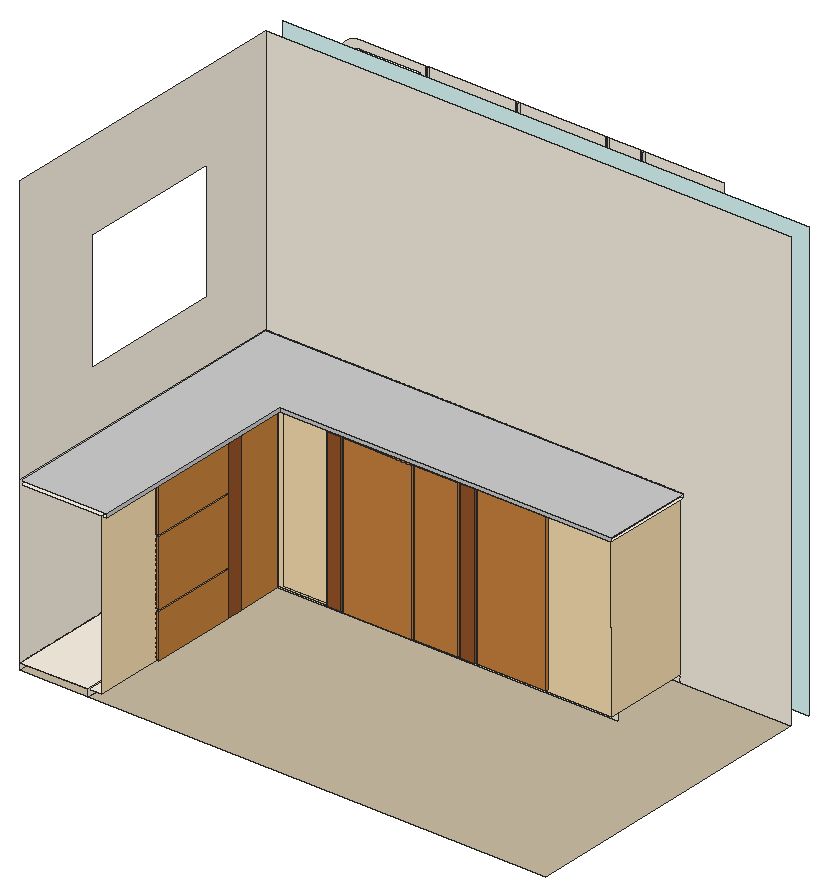
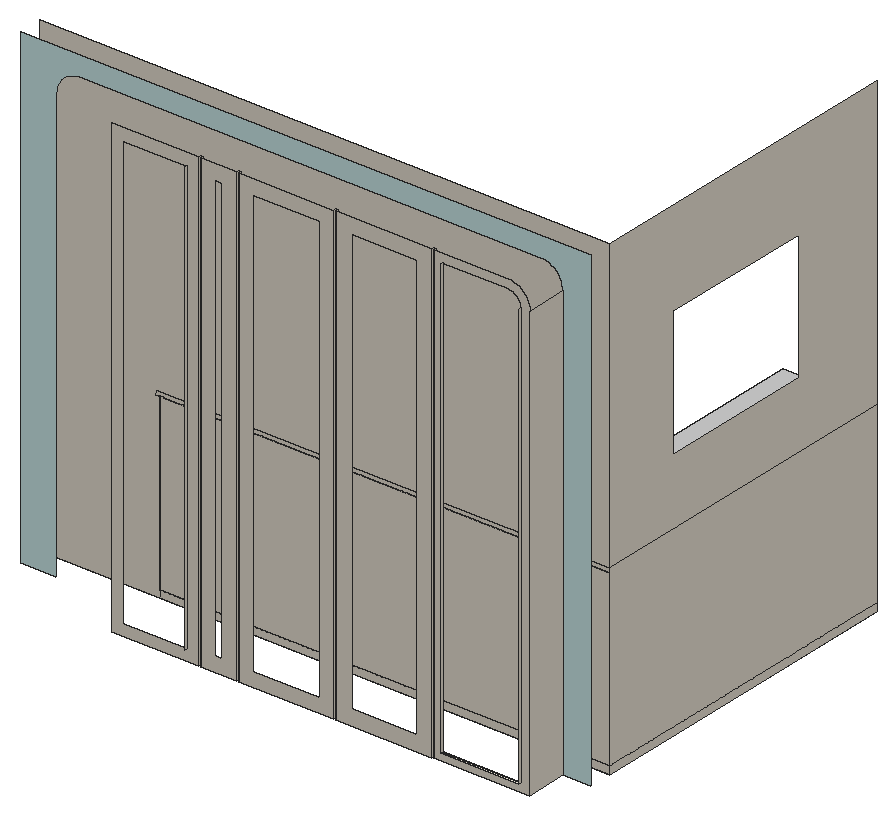
# SketchUp Ruby script. Lengths in inches.
U = 1.inch
M = Sketchup.active_model
def pt(a) = Geom::Point3d.new(a.map { |v| v * U })
def face(e, loops, mat)
  f = e.add_face(loops[0].map { |a| pt(a) })
  loops[1..].each { |l| e.add_face(l.map { |a| pt(a) }).erase! }
  f.material = f.back_material = mat if mat
  f
end
# faces: each face lists its corners as indices into pts; further lists are holes
def faces(e, pts, list, mat = nil) = list.each { |f| face(e, (f[0].is_a?(Array) ? f : [f]).map { |l| l.map { |i| pts[i] } }, mat) }
# xy, xz, yz: faces in a plane at the given z, y or x. An outline is a flat list of corners, or four numbers for a rectangle; further outlines are holes
def ring(l) = l.size == 4 ? [[l[0], l[1]], [l[2], l[1]], [l[2], l[3]], [l[0], l[3]]] : l.each_slice(2).to_a
def flat(e, list, mat, &to3) = list.each { |f| face(e, (f[0].is_a?(Array) ? f : [f]).map { |l| ring(l).map { |u, v| to3.(u, v) } }, mat) }
def xy(e, z, list, mat = nil) = flat(e, list, mat) { |x, y| [x, y, z] }
def xz(e, y, list, mat = nil) = flat(e, list, mat) { |x, z| [x, y, z] }
def yz(e, x, list, mat = nil) = flat(e, list, mat) { |y, z| [x, y, z] }
def lines(e, pts, list) = list.each { |a, b| e.add_line(pt(pts[a]), pt(pts[b])) }
# prism: a flat outline (further loops are holes) pulled along v
def prism(e, loops, v, mat = nil)
  f = face(e, loops, mat); d = Geom::Vector3d.new(v.map { |x| x * U })
  f.pushpull(f.normal.samedirection?(d) ? d.length : -d.length)
end
def box(e, o, s, mat = nil) = prism(e, [[o, [o[0] + s[0], o[1], o[2]], [o[0] + s[0], o[1] + s[1], o[2]], [o[0], o[1] + s[1], o[2]]]], [0, 0, s[2]], mat)
def at(x, y, z, deg = 0) = Geom::Transformation.translation(pt([x, y, z])) * Geom::Transformation.rotation(ORIGIN, Z_AXIS, deg.degrees)
def axes(o, x, y, z) = Geom::Transformation.new([*x, 0, *y, 0, *z, 0, *pt(o).to_a, 1])
def part(name) = M.definitions.add(name)
# library, detail: a bought-in or finely detailed component or shape, given as its bounding box
def library(name, o, s) = part(name).tap { |d| box(d.entities, o, s) }
def detail(e, o, s) = box(e.add_group.entities, o, s)
def put(e, d, t, mat = nil) = e.add_instance(d, t).tap { |i| i.material = mat if mat }
def group(e, t, mat = nil) = e.add_group.tap { |g| g.transformation = t; g.material = mat if mat }.entities
root = M.entities
M.materials.add("[0030_OldLace]").color = [253, 245, 230]
M.materials.add("[0032_Moccasin]").color = [255, 228, 181]
M.materials.add("[0040_Peru]").color = [205, 133, 63]
M.materials.add("[0090_LightCyan]").color = [224, 255, 255]
M.materials.add("[Carrera Marble]").color = [207, 207, 207]
M.materials.add("[Concrete Tile]").color = [203, 190, 164]
M.materials.add("[Wood Cherry Original]").color = [152, 86, 42]
xy(root,1.9375,[[9,301.46,9,385.46,122.59,385.46,122.59,361.96,31.28,361.96,31.28,301.46]],"[0030_OldLace]")
xy(root,2.2,[[18.24,402.03,37.94,402.71]],"[0030_OldLace]")
xy(root,2.4375,[[31.28,319.96,32.22,343.46],[31.28,343.93,32.22,347.96],[31.28,348.43,32.22,360.46],[49.79,360.87,49.78,361.93,68.78,361.96,68.79,360.9],[45.29,360.99,45.28,361.93,49.28,361.96,49.29,361.03],
  [69.29,360.99,69.28,361.93,81.28,361.96,81.29,361.03],[81.79,361.12,81.78,361.93,85.78,361.96,85.79,361.15],[86.29,361.24,86.28,361.93,105.28,361.96,105.29,361.28]],"[0030_OldLace]")
xy(root,14.4375,[[31.28,319.96,32.22,343.46]],"[0040_Peru]")
xy(root,14.9375,[[31.28,319.96,32.22,343.45]],"[0030_OldLace]")
xy(root,32.6875,[[31.28,319.96,32.22,343.45]],"[0040_Peru]")
xy(root,33.1875,[[31.28,319.96,32.22,343.4375]],"[0030_OldLace]")
xy(root,45.1875,[[31.28,319.96,32.22,343.4375],[31.28,348.43,32.22,360.46],[49.79,360.87,68.79,360.9,68.78,361.96,49.78,361.93],[69.29,360.99,81.29,361.03,81.28,361.96,69.28,361.93],[86.29,361.24,105.29,361.28,105.28,361.96,86.28,361.93]],"[0040_Peru]")
xy(root,45.1875,[[31.28,343.93,32.22,347.96],[45.29,360.99,49.29,361.03,49.28,361.96,45.28,361.93],[81.79,361.12,85.79,361.15,85.78,361.96,81.78,361.93]],"[Wood Cherry Original]")
xy(root,45.6875,[[9,301.46,9,385.46,123.52,385.46,123.52,360.6875,32.64,360.6875,32.64,301.46]],"[0030_OldLace]")
xy(root,46.625,[[9,301.46,32.64,301.46,32.64,360.6875,123.52,360.6875,123.52,385.46,9,385.46]],"[Carrera Marble]")
xz(root,319.96,[[31.28,2.4375,32.22,14.4375],[31.28,14.9375,32.22,32.6875],[31.28,33.1875,32.22,45.1875]],"[0040_Peru]")
xz(root,343.4375,[[31.28,33.1875,32.22,45.1875]],"[0030_OldLace]")
xz(root,343.45,[[31.28,14.9375,32.22,32.6875]],"[0030_OldLace]")
xz(root,343.46,[[31.28,2.4375,32.22,14.4375]],"[0030_OldLace]")
xz(root,343.93,[[31.28,2.4375,32.22,45.1875]],"[Wood Cherry Original]")
xz(root,347.96,[[31.28,2.4375,32.22,45.1875]],"[Wood Cherry Original]")
xz(root,348.43,[[31.28,2.4375,32.22,45.1875]],"[0040_Peru]")
xz(root,360.46,[[31.28,2.4375,32.22,45.1875]],"[0030_OldLace]")
xz(root,360.6875,[[32.64,45.6875,123.52,46.625]],"[Carrera Marble]")
xz(root,385.46,[[122.59,0,153,0,153,120,9,120,9,46.625,123.52,46.625,123.52,45.6875,122.59,45.6875],[9,0,122.59,1.9375],[9,1.9375,122.59,45.6875],[9,45.6875,123.52,46.625]],"[0030_OldLace]")
xz(root,391.46,[[9,0,9,120,153,120,153,0,143.9375,0,143.9375,108.93,143.89,109.72,143.73,110.5,143.48,111.25,143.125,111.96,142.68,112.625,142.16,113.22,141.5625,113.74,140.9,114.1875,140.1875,114.54,139.44,114.79,138.66,114.95,137.86,115,21.59,115,20.87,114.95,20.16,114.8125,19.47,114.58,18.82,114.26,18.22,113.85,17.67,113.375,17.19,112.83,16.79,112.23,16.47,111.58,16.24,110.89,16.1,110.18,16.05,109.45,16.05,0]],"[0090_LightCyan]")
xz(root,401.46,[[40.14,0,40.64,115],[64.9,0,65.38,115],[89.38,0,89.9375,115],[99.07,0,99.5625,115]],"[0030_OldLace]")
xz(root,402.03,[[[16.05,0,16.05,109.45,16.1,110.18,16.24,110.89,16.47,111.58,16.79,112.23,17.19,112.83,17.67,113.375,18.22,113.85,18.82,114.26,19.47,114.58,20.16,114.8125,20.87,114.95,21.59,115,40.14,115,40.14,0],[18.24,2.2,37.94,2.2,37.94,112.8,21.59,112.8,21.16,112.78,20.73,112.69,20.3125,112.55,19.92,112.36,19.55,112.11,19.22,111.82,18.9375,111.49,18.69,111.13,18.5,110.74,18.36,110.32,18.27,109.89,18.24,109.45]],[[40.64,0,64.9,115],[44.51,3.87,61.02,111.13]],[[65.38,0,89.38,115],[68.98,3.6,85.78,111.4]],[[89.9375,0,99.07,115],[93.66,3.73,95.34,111.27]],[[99.5625,0,121.45,115],[102.43,2.87,118.59,112.13]]],"[0030_OldLace]")
yz(root,9,[[301.46,0,385.46,1.9375],[301.46,1.9375,385.46,46.625],[[301.46,46.625,385.46,120],[326.03,63.5,365.53,96]]],"[0030_OldLace]")
yz(root,16.05,[[391.46,0,402.03,109.45]],"[0030_OldLace]")
yz(root,18.24,[[402.03,2.2,402.71,109.45]],"[0030_OldLace]")
yz(root,31.28,[[319.96,2.4375,343.46,14.4375],[343.93,2.4375,347.96,45.1875],[348.43,2.4375,360.46,45.1875],[319.96,14.9375,343.45,32.6875],[319.96,33.1875,343.4375,45.1875]],"[0030_OldLace]")
yz(root,32.22,[[319.96,2.4375,343.46,14.4375],[348.43,2.4375,360.46,45.1875],[319.96,14.9375,343.45,32.6875],[319.96,33.1875,343.4375,45.1875]],"[0040_Peru]")
yz(root,32.22,[[343.93,2.4375,347.96,45.1875]],"[Wood Cherry Original]")
yz(root,32.64,[[301.46,45.6875,360.6875,46.625]],"[Carrera Marble]")
yz(root,37.94,[[402.03,2.2,402.71,112.8]],"[0030_OldLace]")
yz(root,40.14,[[401.46,0,402.03,115]],"[0030_OldLace]")
yz(root,40.64,[[401.46,0,402.03,115]],"[0030_OldLace]")
yz(root,64.9,[[401.46,0,402.03,115]],"[0030_OldLace]")
yz(root,65.38,[[401.46,0,402.03,115]],"[0030_OldLace]")
yz(root,89.38,[[401.46,0,402.03,115]],"[0030_OldLace]")
yz(root,89.9375,[[401.46,0,402.03,115]],"[0030_OldLace]")
yz(root,99.07,[[401.46,0,402.03,115]],"[0030_OldLace]")
yz(root,99.5625,[[401.46,0,402.03,115]],"[0030_OldLace]")
yz(root,102.43,[[402.03,2.87,402.71,112.13]],"[0030_OldLace]")
p = [[68.79,360.9,2.4375],[68.79,360.9,45.1875],[49.79,360.87,45.1875],[49.79,360.87,2.4375],[49.78,361.93,45.1875],[49.78,361.93,2.4375],
  [68.78,361.96,2.4375],[68.78,361.96,45.1875],[49.29,361.03,2.4375],[49.29,361.03,45.1875],[45.29,360.99,45.1875],[45.29,360.99,2.4375],
  [45.28,361.93,45.1875],[45.28,361.93,2.4375],[49.28,361.96,2.4375],[49.28,361.96,45.1875],[69.29,360.99,2.4375],[81.29,361.03,2.4375],
  [81.29,361.03,45.1875],[69.29,360.99,45.1875],[69.28,361.93,45.1875],[69.28,361.93,2.4375],[81.28,361.96,2.4375],[81.28,361.96,45.1875],
  [81.79,361.12,45.1875],[81.79,361.12,2.4375],[85.79,361.15,2.4375],[85.79,361.15,45.1875],[81.78,361.93,45.1875],[81.78,361.93,2.4375],
  [85.78,361.96,2.4375],[85.78,361.96,45.1875],[86.29,361.24,45.1875],[86.29,361.24,2.4375],[105.29,361.28,2.4375],[105.29,361.28,45.1875],
  [86.28,361.93,45.1875],[86.28,361.93,2.4375],[105.28,361.96,2.4375],[105.28,361.96,45.1875],[27.65,364.03,0],[27.65,301.46,0],
  [122.59,364.03,0]]
faces(root,p,[[0,1,2,3],[4,5,3,2],[6,7,1,0],[16,17,18,19],[20,21,16,19],[22,23,18,17],[32,33,34,35],[36,37,33,32],
  [38,39,35,34]],"[0040_Peru]")
faces(root,p,[[8,9,10,11],[12,13,11,10],[14,15,9,8],[24,25,26,27],[28,29,25,24],[30,31,27,26]],"[Wood Cherry Original]")
faces(root,p,[[15,14,13,12],[7,6,5,4],[22,21,20,23],[29,28,31,30],[37,36,39,38]],"[0030_OldLace]")
lines(root,p,[[40,41],[40,42]])
g1 = group(root,at(9,301.46,0),"[0030_OldLace]")
xy(g1,1.9375,[[0,0,18.65,0,18.65,62.5625,113.59,62.5625,113.59,84,0,84]])
xz(g1,62.5625,[[18.65,0,113.59,1.9375]])
yz(g1,18.65,[[0,0,62.5625,1.9375]])
g2 = group(root,at(9,301.46,1.9375),"[0030_OldLace]")
xy(g2,43.75,[[0,0,22.28,0,22.28,60.46,113.59,60.46,113.59,84,0,84]],"[0032_Moccasin]")
yz(g2,22.28,[[0,0,60.5,0,60.46,43.75,0,43.75]],"[0032_Moccasin]")
yz(g2,113.59,[[60.5,0,84,0,84,43.75,60.46,43.75]],"[0032_Moccasin]")
p = [[22.28,60.46,43.75],[22.28,60.5,0],[113.59,60.5,0],[113.59,60.46,43.75],[35.78,60.47,43.25],[23.78,60.47,43.25],
  [23.78,60.47,0.5],[35.78,60.5,0.5]]
faces(g2,p,[[0,1,2,3]],"[0032_Moccasin]")
lines(g2,p,[[4,5],[5,6],[6,7],[7,4]])
g3 = group(root,at(9,301.46,0),"[Concrete Tile]")
xy(g3,0,[[0,0,144,84]])
